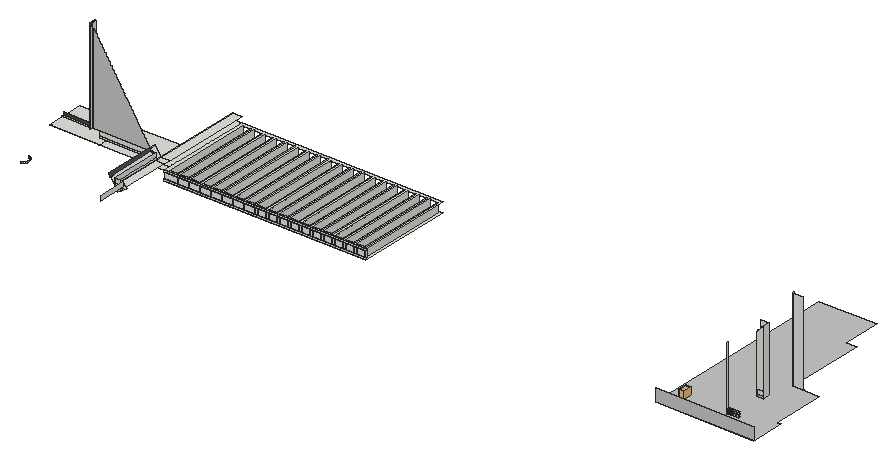
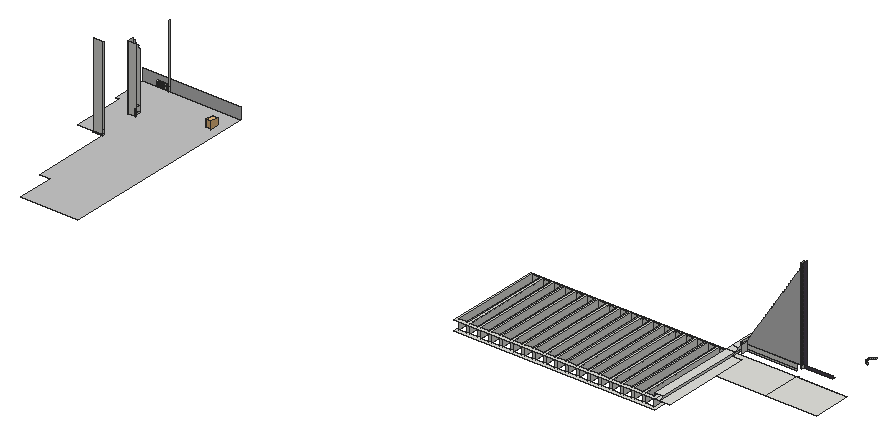
# SketchUp Ruby script. Lengths in inches.
U = 1.inch
M = Sketchup.active_model
def pt(a) = Geom::Point3d.new(a.map { |v| v * U })
def face(e, loops, mat)
  f = e.add_face(loops[0].map { |a| pt(a) })
  loops[1..].each { |l| e.add_face(l.map { |a| pt(a) }).erase! }
  f.material = f.back_material = mat if mat
  f
end
# faces: each face lists its corners as indices into pts; further lists are holes
def faces(e, pts, list, mat = nil) = list.each { |f| face(e, (f[0].is_a?(Array) ? f : [f]).map { |l| l.map { |i| pts[i] } }, mat) }
# xy, xz, yz: faces in a plane at the given z, y or x. An outline is a flat list of corners, or four numbers for a rectangle; further outlines are holes
def ring(l) = l.size == 4 ? [[l[0], l[1]], [l[2], l[1]], [l[2], l[3]], [l[0], l[3]]] : l.each_slice(2).to_a
def flat(e, list, mat, &to3) = list.each { |f| face(e, (f[0].is_a?(Array) ? f : [f]).map { |l| ring(l).map { |u, v| to3.(u, v) } }, mat) }
def xy(e, z, list, mat = nil) = flat(e, list, mat) { |x, y| [x, y, z] }
def xz(e, y, list, mat = nil) = flat(e, list, mat) { |x, z| [x, y, z] }
def yz(e, x, list, mat = nil) = flat(e, list, mat) { |y, z| [x, y, z] }
def lines(e, pts, list) = list.each { |a, b| e.add_line(pt(pts[a]), pt(pts[b])) }
# prism: a flat outline (further loops are holes) pulled along v
def prism(e, loops, v, mat = nil)
  f = face(e, loops, mat); d = Geom::Vector3d.new(v.map { |x| x * U })
  f.pushpull(f.normal.samedirection?(d) ? d.length : -d.length)
end
def box(e, o, s, mat = nil) = prism(e, [[o, [o[0] + s[0], o[1], o[2]], [o[0] + s[0], o[1] + s[1], o[2]], [o[0], o[1] + s[1], o[2]]]], [0, 0, s[2]], mat)
def at(x, y, z, deg = 0) = Geom::Transformation.translation(pt([x, y, z])) * Geom::Transformation.rotation(ORIGIN, Z_AXIS, deg.degrees)
def axes(o, x, y, z) = Geom::Transformation.new([*x, 0, *y, 0, *z, 0, *pt(o).to_a, 1])
def part(name) = M.definitions.add(name)
# library, detail: a bought-in or finely detailed component or shape, given as its bounding box
def library(name, o, s) = part(name).tap { |d| box(d.entities, o, s) }
def detail(e, o, s) = box(e.add_group.entities, o, s)
def put(e, d, t, mat = nil) = e.add_instance(d, t).tap { |i| i.material = mat if mat }
def group(e, t, mat = nil) = e.add_group.tap { |g| g.transformation = t; g.material = mat if mat }.entities
root = M.entities
M.materials.add("[Color M01]").color = [226, 226, 226]
M.materials.add("[Color M02]").color = [198, 198, 198]
M.materials.add("[Color M06]").color = [79, 71, 84]
c1 = library("Group\#13",[0,0,0],[3.54,3.54,3.9375])
xy(root,240.88,[[[686.84,521.5625,901.22,623.84],[889.82,523.31,898.51,620.37],[878.13,523.31,886.82,620.37],[866.44,523.31,875.13,620.37],[854.76,523.31,863.44,620.37],[843.07,523.31,851.76,620.37],[831.38,523.31,840.07,620.37],[819.69,523.31,828.38,620.37],[808.01,523.31,816.69,620.37],[796.32,523.31,805.01,620.37],[784.63,523.31,793.32,620.37],[772.94,523.31,781.63,620.37],[761.26,523.31,769.94,620.37],[749.57,523.31,758.26,620.37],[737.88,523.31,746.57,620.37],[726.19,523.31,734.88,620.37],[714.51,523.31,723.19,620.37],[702.82,523.31,711.51,620.37],[691.13,523.31,699.82,620.37]]])
xy(root,242.34,[[686.84,521.5625,901.22,522.8125]])
xy(root,249.61,[[686.84,521.5625,901.22,522.8125]])
xy(root,251.0625,[[565.03,521.5625,618.43,562.32],[618.43,521.5625,618.43,562.32,671.33,562.32,671.33,527.76,686.84,527.76,686.84,521.5625],[[686.84,521.5625,901.22,623.84],[889.82,523.31,898.51,620.37],[878.13,523.31,886.82,620.37],[866.44,523.31,875.13,620.37],[854.76,523.31,863.44,620.37],[843.07,523.31,851.76,620.37],[831.38,523.31,840.07,620.37],[819.69,523.31,828.38,620.37],[808.01,523.31,816.69,620.37],[796.32,523.31,805.01,620.37],[784.63,523.31,793.32,620.37],[772.94,523.31,781.63,620.37],[761.26,523.31,769.94,620.37],[749.57,523.31,758.26,620.37],[737.88,523.31,746.57,620.37],[726.19,523.31,734.88,620.37],[714.51,523.31,723.19,620.37],[702.82,523.31,711.51,620.37],[691.13,523.31,699.82,620.37]],[671.33,527.76,686.84,623.84],[1322.24,561.375,1333.06,562.32]])
xy(root,251.0625,[[1249.48,469.875,1249.48,686.3125,1310.86,686.3125,1310.86,646.3125,1322.24,646.3125,1322.24,561.375,1350.1,561.375,1350.1,505.3125,1354.48,505.3125,1354.48,469.875]],"[Color M02]")
xy(root,257.0625,[[677.53,467.1875,686.84,521.5625],[677.53,521.5625,686.84,528.48],[1316.04,521.5625,1322.24,528.48],[1322.24,521.5625,1322.96,528.48],[677.53,528.48,686.84,623.84]])
xy(root,259.68,[[1319.2,480.14,1321.51,480.77],[1322.11,480.14,1324.42,480.77],[1325.02,480.14,1327.33,480.77],[1327.93,480.14,1330.25,480.77]])
xy(root,262,[[1319.2,480.14,1321.51,480.77],[1322.11,480.14,1324.42,480.77],[1325.02,480.14,1327.33,480.77],[1327.93,480.14,1330.25,480.77]])
xy(root,262.73,[[1319.23,480.14,1321.54,480.77],[1322.14,480.14,1324.45,480.77],[1325.05,480.14,1327.36,480.77],[1327.96,480.14,1330.28,480.77]])
xy(root,263.89,[[609.02,519.6875,610.9,521.5625],[578.05,521.5625,609.02,523.75],[609.02,521.5625,610.9,526.125]])
xy(root,265.04,[[1319.23,480.14,1321.54,480.77],[1322.14,480.14,1324.45,480.77],[1325.05,480.14,1327.36,480.77],[1327.96,480.14,1330.28,480.77]])
xz(root,467.1875,[[680.77,252.01,684.82,254.61,683.25,257.0625,677.53,257.0625],[684.82,254.61,690.08,257.98,686.84,263.03,686.84,257.0625,683.25,257.0625],[677.53,257.0625,683.25,258.95],[683.25,257.0625,686.84,258.95],[677.53,258.95,683.25,263.89],
  [683.25,258.95,686.84,258.95,686.84,263.03,686.29,263.89,683.25,263.89],[686.84,263.03,686.29,263.89,686.84,263.89]])
xz(root,469.875,[[1249.48,251.0625,1354.48,263.89]],"[Color M02]")
xz(root,480.14,[[1317.4375,258.95,1318.58,263.89],[1319.23,262.73,1321.54,263.89],[1322.14,262.73,1324.45,263.89],[1325.05,262.73,1327.36,263.89],[1327.96,262.73,1330.28,263.89]])
xz(root,480.77,[[1319.23,262.73,1321.54,263.89],[1322.14,262.73,1324.45,263.89],[1325.05,262.73,1327.36,263.89]])
xz(root,519.6875,[[609.02,263.89,610.9,263.89,610.9,360.99,610.53,360.76,610.47,360.85,610.84,361.08,610.21,362.07,609.84,361.83,609.02,363.11]],"[Color M06]")
xz(root,521.5625,[[686.84,240.88,901.22,242.34],[686.84,249.61,901.22,251.0625],[565.03,250.875,618.43,251.0625],[618.43,257.0625,671.46,258.95],[671.46,257.0625,677.53,257.0625,676.32,258.95,671.46,258.95],
  [677.53,257.0625,676.32,258.95,677.53,258.95],[1316.04,257.0625,1322.96,258.95],[618.43,258.95,671.46,263.89],[671.46,258.95,676.32,258.95,673.15,263.89,672.89,263.72,672.78,263.89,671.46,263.89],[676.32,258.95,673.15,263.89,676.32,263.89],
  [676.32,258.95,677.53,263.89],[1316.04,258.95,1322.96,263.89],[672.89,263.72,672.78,263.89,673.15,263.89],[671.46,263.89,672.78,263.89,671.46,265.95],[672.78,263.89,673.15,263.89,671.46,266.53,671.46,265.95],
  [1316.04,263.89,1322.96,263.89,1322.96,325.17,1322.03,324.17,1321.57,324.6,1320.69,323.67,1321.15,323.24,1318.73,320.67,1318.27,321.1,1317.39,320.17,1317.85,319.74,1316.5,318.3,1316.04,317.82]])
xz(root,521.5625,[[610.9,263.89,671.46,263.89,671.46,265.95,671.2,266.36,671.46,266.53,670.93,267.36,670.66,267.19,668.97,269.84,669.23,270,668.7,270.83,668.4375,270.67,666.74,273.31,667.01,273.48,666.47,274.31,666.21,274.14,664.52,276.78,664.78,276.95,664.25,277.78,663.98,277.61,662.29,280.25,662.55,280.42,662.02,281.25,661.76,281.08,660.0625,283.73,660.33,283.89,659.8,284.72,659.53,284.56,657.84,287.2,658.1,287.37,657.57,288.2,657.31,288.03,655.61,290.67,655.875,290.84,655.34,291.67,655.08,291.5,653.39,294.14,653.65,294.3125,653.12,295.14,652.85,294.97,651.16,297.62,651.42,297.79,650.89,298.61,650.625,298.45,648.93,301.09,649.2,301.26,648.66,302.09,648.3,301.85,646.6,304.49,646.97,304.73,646.4375,305.56,646.07,305.32,644.375,307.97,644.74,308.2,644.21,309.03,643.84,308.8,642.15,311.44,642.52,311.68,641.98,312.51,641.62,312.27,639.92,314.91,640.29,315.15,639.76,315.98,639.39,315.74,637.7,318.38,638.0625,318.62,637.53,319.45,637.16,319.21,635.47,321.86,635.84,322.09,635.31,322.92,634.9375,322.6875,633.24,325.33,633.61,325.57,633.08,326.4,632.71,326.16,631.02,328.8,631.39,329.04,630.85,329.87,630.48,329.63,628.79,332.28,629.16,332.51,628.625,333.34,628.26,333.11,626.5625,335.75,626.93,335.98,626.4,336.8125,626.03,336.58,624.34,339.22,624.71,339.46,624.28,340.125,624.17,340.29,623.81,340.05,622.11,342.69,622.48,342.93,621.85,343.92,621.48,343.68,619.78,346.32,620.15,346.56,619.52,347.55,619.15,347.3125,617.46,349.95,617.82,350.19,617.19,351.18,616.82,350.94,615.13,353.58,615.5,353.82,614.86,354.81,614.5,354.57,612.8,357.22,613.17,357.45,612.54,358.4375,612.17,358.2,610.9,360.18]],"[Color M02]")
xz(root,522.8125,[[686.84,242.34,901.22,249.61]],"[Color M01]")
xz(root,523.31,[[691.13,240.88,699.82,251.0625],[702.82,240.88,711.51,251.0625],[714.51,240.88,723.19,251.0625],[726.19,240.88,734.88,251.0625],[737.88,240.88,746.57,251.0625],
  [749.57,240.88,758.26,251.0625],[761.26,240.88,769.94,251.0625],[772.94,240.88,781.63,251.0625],[784.63,240.88,793.32,251.0625],[796.32,240.88,805.01,251.0625],
  [808.01,240.88,816.69,251.0625],[819.69,240.88,828.38,251.0625],[831.38,240.88,840.07,251.0625],[843.07,240.88,851.76,251.0625],[854.76,240.88,863.44,251.0625],
  [866.44,240.88,875.13,251.0625],[878.13,240.88,886.82,251.0625],[889.82,240.88,898.51,251.0625]])
xz(root,523.75,[[578.05,263.89,609.02,267.02]],"[Color M06]")
xz(root,526.125,[[609.02,263.89,610.9,363.92]])
xz(root,528.48,[[1314.46,257.0625,1316.04,258.95],[1316.04,257.0625,1322.96,257.0625,1322.96,326.08,1314.46,326.08,1314.46,263.89,1316.04,263.89],[1314.46,258.95,1316.04,263.89]])
xz(root,561.375,[[1322.24,251.0625,1333.06,340.125]])
yz(root,609.02,[[523.75,263.89,526.125,267.02]])
yz(root,609.02,[[519.6875,263.89,519.6875,363.92,524.25,363.92,524.25,362,526.125,362,526.125,361.18,524.25,361.18,524.25,358.06,526.125,358.06,526.125,357.25,524.25,357.25,524.25,354.12,526.125,354.12,526.125,353.18,524.25,353.18,524.25,350.06,526.125,350.06,526.125,349.12,524.25,349.12,524.25,346,526.125,346,526.125,345.06,524.25,345.06,524.25,341.93,526.125,341.93,526.125,341.52,524.25,341.52,524.25,338.39,526.125,338.39,526.125,337.64,524.25,337.64,524.25,334.51,526.125,334.51,526.125,333.77,524.25,333.77,524.25,330.64,526.125,330.64,526.125,329.89,524.25,329.89,524.25,326.76,526.125,326.76,526.125,326.02,524.25,326.02,524.25,322.89,526.125,322.89,526.125,322.14,524.25,322.14,524.25,319.01,526.125,319.01,526.125,318.2,524.25,318.2,524.25,315.08,526.125,315.08,526.125,314.27,523.75,314.27,523.75,311.14,526.125,311.14,526.125,310.33,523.75,310.33,523.75,307.2,526.125,307.2,526.125,306.39,523.75,306.39,523.75,303.26,526.125,303.26,526.125,302.45,523.75,302.45,523.75,299.33,526.125,299.33,526.125,298.52,523.75,298.52,523.75,295.39,526.125,295.39,526.125,294.58,523.75,294.58,523.75,291.45,526.125,291.45,526.125,290.64,523.75,290.64,523.75,287.51,526.125,287.51,526.125,286.7,523.75,286.7,523.75,283.58,526.125,283.58,526.125,282.77,523.75,282.77,523.75,279.64,526.125,279.64,526.125,278.83,523.75,278.83,523.75,275.7,526.125,275.7,526.125,274.89,523.75,274.89,523.75,271.76,526.125,271.76,526.125,270.95,523.75,270.95,523.75,267.83,526.125,267.83,526.125,267.02,523.75,267.02,523.75,263.89]],"[Color M06]")
yz(root,610.9,[[519.6875,263.89,521.5625,360.99],[521.5625,263.89,526.125,363.92]])
yz(root,671.46,[[521.5625,257.0625,528.48,266.53]])
yz(root,677.53,[[467.1875,257.0625,521.5625,258.95],[467.1875,258.95,521.5625,263.89]])
yz(root,686.84,[[437.0625,258.95,467.1875,263.89]])
yz(root,691.13,[[523.31,240.88,620.37,251.0625]])
yz(root,699.82,[[523.31,240.88,620.37,251.0625]])
yz(root,702.82,[[523.31,240.88,620.37,251.0625]])
yz(root,711.51,[[523.31,240.88,620.37,251.0625]])
yz(root,714.51,[[523.31,240.88,620.37,251.0625]])
yz(root,723.19,[[523.31,240.88,620.37,251.0625]])
yz(root,726.19,[[523.31,240.88,620.37,251.0625]])
yz(root,734.88,[[523.31,240.88,620.37,251.0625]])
yz(root,737.88,[[523.31,240.88,620.37,251.0625]])
yz(root,746.57,[[523.31,240.88,620.37,251.0625]])
yz(root,749.57,[[523.31,240.88,620.37,251.0625]])
yz(root,758.26,[[523.31,240.88,620.37,251.0625]])
yz(root,761.26,[[523.31,240.88,620.37,251.0625]])
yz(root,769.94,[[523.31,240.88,620.37,251.0625]])
yz(root,772.94,[[523.31,240.88,620.37,251.0625]])
yz(root,781.63,[[523.31,240.88,620.37,251.0625]])
yz(root,784.63,[[523.31,240.88,620.37,251.0625]])
yz(root,793.32,[[523.31,240.88,620.37,251.0625]])
yz(root,796.32,[[523.31,240.88,620.37,251.0625]])
yz(root,805.01,[[523.31,240.88,620.37,251.0625]])
yz(root,808.01,[[523.31,240.88,620.37,251.0625]])
yz(root,816.69,[[523.31,240.88,620.37,251.0625]])
yz(root,819.69,[[523.31,240.88,620.37,251.0625]])
yz(root,828.38,[[523.31,240.88,620.37,251.0625]])
yz(root,831.38,[[523.31,240.88,620.37,251.0625]])
yz(root,840.07,[[523.31,240.88,620.37,251.0625]])
yz(root,843.07,[[523.31,240.88,620.37,251.0625]])
yz(root,851.76,[[523.31,240.88,620.37,251.0625]])
yz(root,854.76,[[523.31,240.88,620.37,251.0625]])
yz(root,863.44,[[523.31,240.88,620.37,251.0625]])
yz(root,866.44,[[523.31,240.88,620.37,251.0625]])
yz(root,875.13,[[523.31,240.88,620.37,251.0625]])
yz(root,878.13,[[523.31,240.88,620.37,251.0625]])
yz(root,886.82,[[523.31,240.88,620.37,251.0625]])
yz(root,889.82,[[523.31,240.88,620.37,251.0625]])
yz(root,898.51,[[523.31,240.88,620.37,251.0625]])
yz(root,1316.04,[[521.5625,257.0625,528.48,258.95],[521.5625,258.95,528.48,263.89]])
yz(root,1317.4375,[[480.14,258.95,480.77,263.89],[480.14,263.89,480.77,326.5]])
yz(root,1319.2,[[480.14,259.68,480.77,262]])
yz(root,1319.23,[[480.14,262.73,480.77,265.04]])
yz(root,1321.51,[[480.14,259.68,480.77,262]])
yz(root,1321.54,[[480.14,262.73,480.77,265.04]])
yz(root,1322.11,[[480.14,259.68,480.77,262]])
yz(root,1322.14,[[480.14,262.73,480.77,265.04]])
yz(root,1322.24,[[561.375,251.0625,562.32,253.4375],[561.375,253.4375,562.32,257.0625],[561.375,257.0625,562.32,340.125]])
yz(root,1322.96,[[521.5625,257.0625,528.48,326.08]])
yz(root,1324.42,[[480.14,259.68,480.77,262]])
yz(root,1324.45,[[480.14,262.73,480.77,265.04]])
yz(root,1325.02,[[480.14,259.68,480.77,262]])
yz(root,1325.05,[[480.14,262.73,480.77,265.04]])
yz(root,1327.33,[[480.14,259.68,480.77,262]])
yz(root,1327.36,[[480.14,262.73,480.77,265.04]])
yz(root,1327.93,[[480.14,259.68,480.77,262]])
yz(root,1327.96,[[480.14,262.73,480.77,265.04]])
p = [[587.46,457.2,250.875],[586.02,456.6,250.875],[586.02,456.6,252.25],[587.46,457.2,252.25],[588.71,458.15,250.875],[588.71,458.15,252.25],
  [589.66,459.39,250.875],[589.66,459.39,252.25],[590.26,460.84,250.875],[590.26,460.84,252.25],[590.46,462.39,250.875],[590.46,462.39,252.25],
  [590.26,463.95,250.875],[590.26,463.95,252.25],[589.66,465.39,250.875],[589.66,465.39,252.25],[588.71,466.64,250.875],[588.71,466.64,252.25],
  [587.46,467.59,250.875],[587.46,467.59,252.25],[586.02,468.1875,250.875],[586.02,468.1875,252.25],[677.53,467.1875,257.0625],[677.53,521.5625,257.0625],
  [680.77,521.5625,252.01],[680.77,467.1875,252.01],[677.53,528.48,257.0625],[680.77,528.48,252.01],[677.53,623.84,257.0625],[680.77,623.84,252.01],
  [673.15,467.1875,263.89],[673.15,521.5625,263.89],[676.32,521.5625,258.95],[671.46,528.48,266.53],[671.46,521.5625,266.53],[671.2,521.5625,266.36],
  [671.46,521.5625,265.95],[672.78,521.5625,263.89],[672.89,521.5625,263.72],[672.89,467.1875,263.72],[671.2,467.1875,266.36],[1316.04,561.375,240.47],
  [1322.24,561.375,240.47],[1322.24,521.5625,251.0625],[1322.24,521.5625,257.0625],[1322.24,562.32,240.47],[1316.04,541.0625,251.0625],[1316.04,541.0625,253.4375]]
faces(root,p,[[0,1,2,3],[4,0,3,5],[6,4,5,7],[8,6,7,9],[10,8,9,11],[12,10,11,13],[14,12,13,15],[16,14,15,17],
  [18,16,17,19],[20,18,19,21],[22,23,24,25],[23,26,27,24],[26,28,29,27],[22,30,31,32,23],[26,33,34,31,32,23],[31,30,39,38]])
faces(root,p,[[35,36,37,38,39,40]],"[Color M06]")
lines(root,p,[[41,42],[43,44],[42,45],[46,47]])
put(root,c1,axes([1265.03,488.625,258.17],[-1.5535,0,0],[0,2.39,0],[0,0,-3.63878]))
